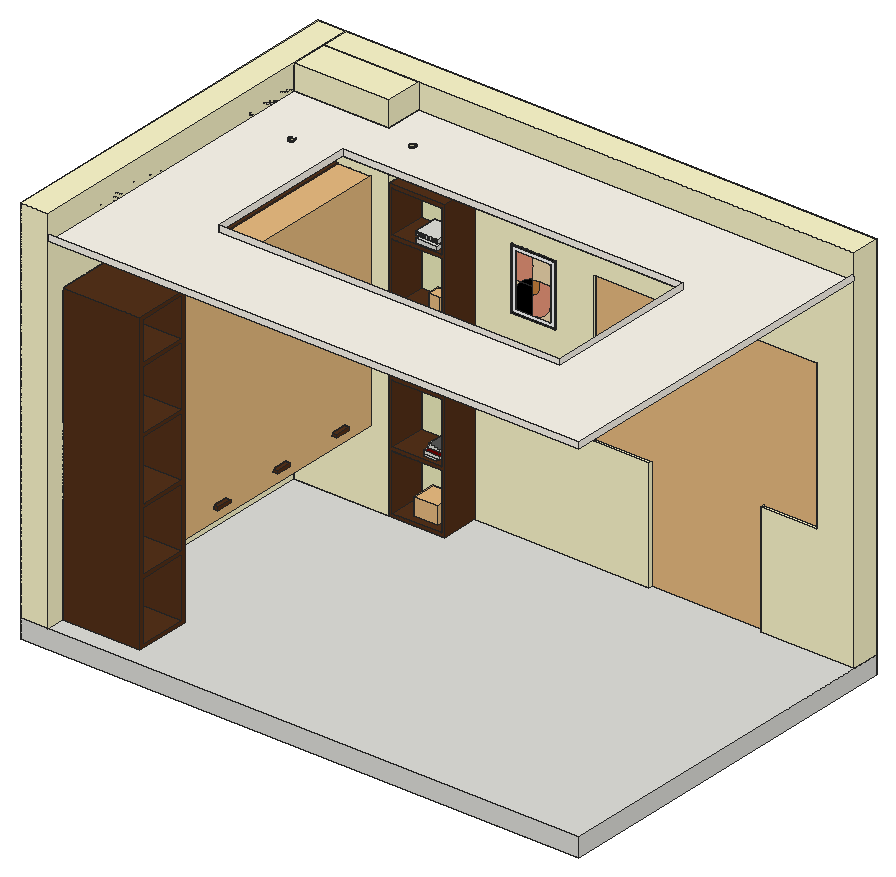
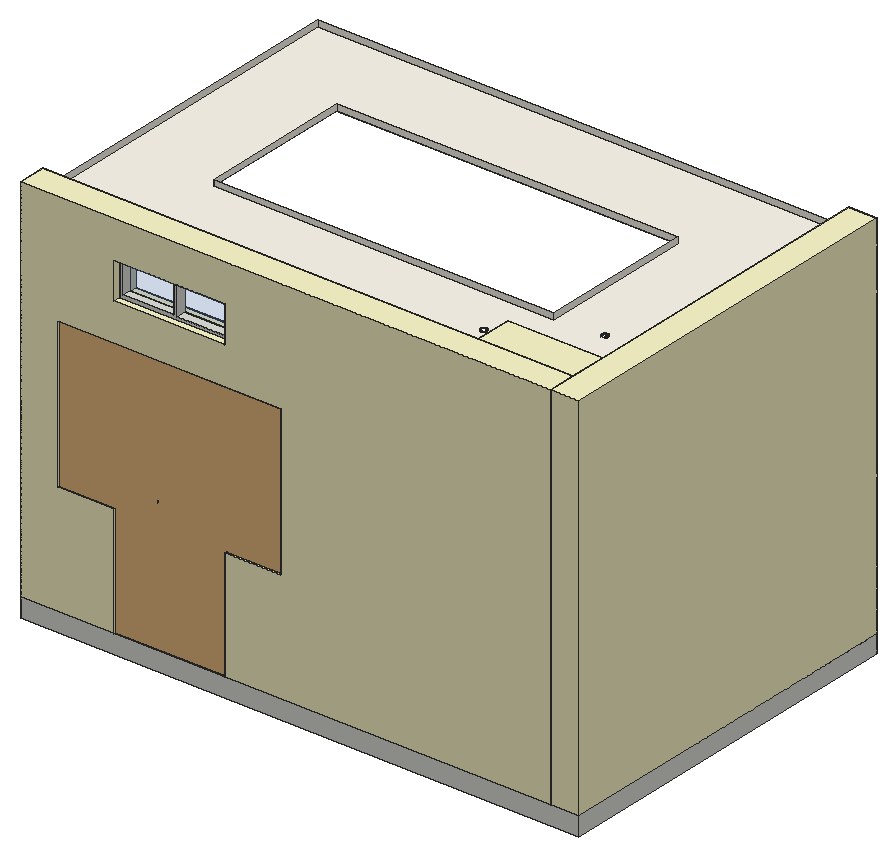
# SketchUp Ruby script. Lengths in inches.
U = 1.inch
M = Sketchup.active_model
def pt(a) = Geom::Point3d.new(a.map { |v| v * U })
def face(e, loops, mat)
  f = e.add_face(loops[0].map { |a| pt(a) })
  loops[1..].each { |l| e.add_face(l.map { |a| pt(a) }).erase! }
  f.material = f.back_material = mat if mat
  f
end
# faces: each face lists its corners as indices into pts; further lists are holes
def faces(e, pts, list, mat = nil) = list.each { |f| face(e, (f[0].is_a?(Array) ? f : [f]).map { |l| l.map { |i| pts[i] } }, mat) }
# xy, xz, yz: faces in a plane at the given z, y or x. An outline is a flat list of corners, or four numbers for a rectangle; further outlines are holes
def ring(l) = l.size == 4 ? [[l[0], l[1]], [l[2], l[1]], [l[2], l[3]], [l[0], l[3]]] : l.each_slice(2).to_a
def flat(e, list, mat, &to3) = list.each { |f| face(e, (f[0].is_a?(Array) ? f : [f]).map { |l| ring(l).map { |u, v| to3.(u, v) } }, mat) }
def xy(e, z, list, mat = nil) = flat(e, list, mat) { |x, y| [x, y, z] }
def xz(e, y, list, mat = nil) = flat(e, list, mat) { |x, z| [x, y, z] }
def yz(e, x, list, mat = nil) = flat(e, list, mat) { |y, z| [x, y, z] }
def lines(e, pts, list) = list.each { |a, b| e.add_line(pt(pts[a]), pt(pts[b])) }
# prism: a flat outline (further loops are holes) pulled along v
def prism(e, loops, v, mat = nil)
  f = face(e, loops, mat); d = Geom::Vector3d.new(v.map { |x| x * U })
  f.pushpull(f.normal.samedirection?(d) ? d.length : -d.length)
end
def box(e, o, s, mat = nil) = prism(e, [[o, [o[0] + s[0], o[1], o[2]], [o[0] + s[0], o[1] + s[1], o[2]], [o[0], o[1] + s[1], o[2]]]], [0, 0, s[2]], mat)
def at(x, y, z, deg = 0) = Geom::Transformation.translation(pt([x, y, z])) * Geom::Transformation.rotation(ORIGIN, Z_AXIS, deg.degrees)
def axes(o, x, y, z) = Geom::Transformation.new([*x, 0, *y, 0, *z, 0, *pt(o).to_a, 1])
def part(name) = M.definitions.add(name)
# library, detail: a bought-in or finely detailed component or shape, given as its bounding box
def library(name, o, s) = part(name).tap { |d| box(d.entities, o, s) }
def detail(e, o, s) = box(e.add_group.entities, o, s)
def put(e, d, t, mat = nil) = e.add_instance(d, t).tap { |i| i.material = mat if mat }
def group(e, t, mat = nil) = e.add_group.tap { |g| g.transformation = t; g.material = mat if mat }.entities
root = M.entities
M.materials.add("[0014_DarkSalmon]").color = [233, 150, 122]
M.materials.add("[0034_Wheat]").color = [245, 222, 179]
M.materials.add("[0040_Peru]").color = [205, 133, 63]
M.materials.add("[0050_LemonChiffon]").color = [255, 250, 205]
M.materials.add("[0052_FloralWhite]").color = [255, 250, 240]
M.materials.add("[0137_Black]").color = [0, 0, 0]
M.materials.add("[Color A08]").color = [102, 0, 0]
M.materials.add("[Color D02]").color = [214, 192, 128]
M.materials.add("[Color D07]").color = [153, 114, 0]
M.materials.add("[Color E01]").color = [242, 242, 193]
M.materials.add("[Color E01]1").color = [255, 255, 204]
M.materials.add("[Color L16]").color = [102, 0, 51]
M.materials.add("[Color M00]").color = [255, 255, 255]
M.materials.add("[Color M06]").color = [86, 86, 86]
M.materials.add("[Color M07]").color = [58, 58, 58]
M.materials.add("[Color M09]").color = [0, 0, 0]
M.materials.add("[Metal Aluminum Anodized]").color = [202, 209, 219]
M.materials.add("[Translucent Glass Blue]").color = [107, 160, 255]
M.materials["[Translucent Glass Blue]"].alpha = 0.26
M.materials.add("[Translucent Glass Gray]").color = [128, 128, 128]
M.materials["[Translucent Glass Gray]"].alpha = 0.5
M.materials.add("[Wood Veneer 01]").color = [112, 65, 34]
M.materials.add("[Wood Veneer 01]1").color = [84, 49, 25]
c1 = library("Group\#12",[0,0,0],[72,7.3,84])
c2 = library("Group\#45",[0,0,0],[7.625,7.62,5.4375])
c3 = library("Group\#23",[2,0,0],[22.8,75,72])
c4 = part("Group\#31")
box(c4.entities,[0,0,0],[1.5,4.9375,1])
c5 = part("Group\#28")
box(c5.entities,[0,0,0],[1,1.53,44.5])
c6 = library("Group\#50",[0,0,0],[5.875,5.87,4.8125])
c7 = library("Group\#49",[0,0,0],[3.75,3.75,5.1875])
c8 = part("Group\#30")
box(c8.entities,[0,0,0],[1,0.5625,2.125])
box(root,[40.6,110.9,7],[16,0.1,94],"[Color E01]")
xy(root,118,[[[9,0,180,111],[39.6,30.6,149.4,80.4],[24.3,77.95,24.37,77.96,24.4375,77.96,24.51,77.98,24.58,77.99,24.64,78.01,24.71,78.04,24.77,78.07,24.83,78.11,24.89,78.14,24.94,78.1875,24.99,78.23,25.04,78.28,25.09,78.34,25.13,78.39,25.17,78.45,25.2,78.52,25.23,78.58,25.25,78.64,25.27,78.71,25.3,78.92,25.3,78.99,25.27,79.2,25.25,79.26,25.23,79.33,25.17,79.45,25.09,79.57,24.94,79.72,24.89,79.76,24.77,79.84,24.71,79.87,24.64,79.89,24.58,79.92,24.51,79.93,24.4375,79.94,24.37,79.95,24.23,79.95,24.02,79.92,23.96,79.89,23.89,79.87,23.83,79.84,23.71,79.76,23.66,79.72,23.51,79.57,23.43,79.45,23.37,79.33,23.35,79.26,23.33,79.2,23.3,78.99,23.3,78.92,23.33,78.71,23.35,78.64,23.37,78.58,23.4,78.52,23.43,78.45,23.47,78.39,23.51,78.34,23.56,78.28,23.61,78.23,23.66,78.1875,23.71,78.14,23.77,78.11,23.83,78.07,23.89,78.04,23.96,78.01,24.02,77.99,24.09,77.98,24.16,77.96,24.23,77.96],[49.94,94.53,50.15,94.53,50.29,94.55,50.36,94.5625,50.42,94.59,50.49,94.61,50.55,94.64,50.67,94.72,50.72,94.76,50.78,94.81,50.82,94.86,50.87,94.91,50.95,95.03,51.01,95.15,51.05,95.29,51.0625,95.35,51.07,95.42,51.08,95.49,51.08,95.5625,51.07,95.63,51.0625,95.7,51.05,95.77,51.03,95.84,51.01,95.9,50.98,95.97,50.94,96.03,50.91,96.09,50.87,96.14,50.82,96.2,50.77,96.25,50.72,96.29,50.66,96.34,50.61,96.375,50.55,96.41,50.48,96.44,50.42,96.47,50.35,96.49,50.28,96.5,50.22,96.52,50.01,96.52,49.9375,96.51,49.87,96.5,49.8,96.49,49.73,96.46,49.67,96.4375,49.61,96.41,49.43,96.29,49.33,96.19,49.29,96.14,49.21,96.02,49.15,95.9,49.11,95.76,49.09,95.7,49.08,95.63,49.08,95.42,49.09,95.35,49.13,95.21,49.15,95.15,49.18,95.08,49.21,95.02,49.25,94.96,49.29,94.91,49.34,94.85,49.39,94.8,49.4375,94.76,49.49,94.71,49.55,94.68,49.61,94.64,49.67,94.61,49.74,94.58,49.81,94.5625,49.875,94.55]]],"[0052_FloralWhite]")
xz(root,0,[[9,118,180,120]],"[0052_FloralWhite]")
xz(root,30.6,[[39.6,118,149.4,120]],"[0052_FloralWhite]")
xz(root,77.96,[[24.16,118,24.23,118.3],[24.37,118,24.4375,118.3]],"[Metal Aluminum Anodized]")
xz(root,80.4,[[39.6,118,149.4,120]],"[0052_FloralWhite]")
xz(root,94.53,[[49.94,118,50.01,118.125],[50.01,118,50.08,118.125],[50.08,118,50.15,118.125]],"[Metal Aluminum Anodized]")
xz(root,96.52,[[50.01,118,50.08,118.125],[50.08,118,50.15,118.125],[50.15,118,50.22,118.125]],"[Metal Aluminum Anodized]")
xz(root,114.5,[[115,103,131.5,113],[132.5,103,149,113]],"[Translucent Glass Blue]")
yz(root,9,[[0,118,111,120]],"[0052_FloralWhite]")
yz(root,23,[[82,40,98,101],[24.5,84.5,33.8125,101.5]],"[Translucent Glass Gray]")
yz(root,23.3,[[78.92,118,78.99,118.3]],"[Metal Aluminum Anodized]")
yz(root,25.3,[[78.92,118,78.99,118.3]],"[Metal Aluminum Anodized]")
yz(root,39.6,[[30.6,118,80.4,120]],"[0052_FloralWhite]")
yz(root,49.08,[[95.42,118,95.49,118.125],[95.49,118,95.56,118.125],[95.56,118,95.63,118.125]],"[Metal Aluminum Anodized]")
yz(root,51.08,[[95.49,118,95.5625,118.125]],"[Metal Aluminum Anodized]")
yz(root,149.4,[[30.6,118,80.4,120]],"[0052_FloralWhite]")
yz(root,180,[[0,118,111,120]],"[0052_FloralWhite]")
p = [[23.89,78.04,118],[23.83,78.07,118],[23.83,78.07,118.3],[23.89,78.04,118.3],[23.96,78.01,118],[23.96,78.01,118.3],
  [24.09,77.98,118],[24.02,77.99,118],[24.02,77.99,118.3],[24.09,77.98,118.3],[24.16,77.96,118],[24.16,77.96,118.3],
  [24.3,77.95,118],[24.23,77.96,118],[24.23,77.96,118.3],[24.3,77.95,118.3],[24.37,77.96,118],[24.37,77.96,118.3],
  [24.51,77.98,118],[24.4375,77.96,118],[24.4375,77.96,118.3],[24.51,77.98,118.3],[24.58,77.99,118],[24.58,77.99,118.3],
  [24.71,78.04,118],[24.64,78.01,118],[24.64,78.01,118.3],[24.71,78.04,118.3],[24.77,78.07,118],[24.77,78.07,118.3],
  [23.77,78.11,118],[23.71,78.14,118],[23.71,78.14,118.3],[23.77,78.11,118.3],[23.66,78.1875,118],[23.66,78.1875,118.3],
  [24.89,78.14,118],[24.83,78.11,118],[24.83,78.11,118.3],[24.89,78.14,118.3],[24.94,78.1875,118],[24.94,78.1875,118.3],
  [23.61,78.23,118],[23.61,78.23,118.3],[23.56,78.28,118],[23.56,78.28,118.3],[24.99,78.23,118],[24.99,78.23,118.3],
  [25.04,78.28,118],[25.04,78.28,118.3],[23.51,78.34,118],[23.51,78.34,118.3],[23.47,78.39,118],[23.47,78.39,118.3],
  [25.09,78.34,118],[25.09,78.34,118.3],[25.13,78.39,118],[25.13,78.39,118.3],[23.43,78.45,118],[23.43,78.45,118.3],
  [25.17,78.45,118],[25.17,78.45,118.3],[23.4,78.52,118],[23.4,78.52,118.3],[23.37,78.58,118],[23.37,78.58,118.3],
  [25.23,78.58,118],[25.2,78.52,118],[25.2,78.52,118.3],[25.23,78.58,118.3],[23.35,78.64,118],[23.35,78.64,118.3],
  [23.33,78.71,118],[23.33,78.71,118.3],[25.25,78.64,118],[25.25,78.64,118.3],[25.27,78.71,118],[25.27,78.71,118.3],
  [23.32,78.78,118],[23.32,78.78,118.3],[25.28,78.78,118],[25.28,78.78,118.3],[23.31,78.85,118],[23.31,78.85,118.3],
  [23.3,78.92,118],[23.3,78.92,118.3],[25.3,78.92,118],[25.29,78.85,118],[25.29,78.85,118.3],[25.3,78.92,118.3],
  [23.3,78.99,118],[23.31,79.06,118],[23.31,79.06,118.3],[23.3,78.99,118.3],[25.29,79.06,118],[25.3,78.99,118],
  [25.3,78.99,118.3],[25.29,79.06,118.3],[23.32,79.13,118],[23.32,79.13,118.3],[23.33,79.2,118],[23.33,79.2,118.3],
  [25.27,79.2,118],[25.28,79.13,118],[25.28,79.13,118.3],[25.27,79.2,118.3],[23.35,79.26,118],[23.35,79.26,118.3],
  [25.25,79.26,118],[25.25,79.26,118.3],[23.37,79.33,118],[23.37,79.33,118.3],[23.4,79.39,118],[23.4,79.39,118.3],
  [25.2,79.39,118],[25.23,79.33,118],[25.23,79.33,118.3],[25.2,79.39,118.3],[23.43,79.45,118],[23.43,79.45,118.3],
  [25.17,79.45,118],[25.17,79.45,118.3],[23.47,79.51,118],[23.47,79.51,118.3],[23.51,79.57,118],[23.51,79.57,118.3],
  [25.09,79.57,118],[25.13,79.51,118],[25.13,79.51,118.3],[25.09,79.57,118.3],[23.56,79.62,118],[23.56,79.62,118.3],
  [23.61,79.67,118],[23.61,79.67,118.3],[24.99,79.67,118],[25.04,79.62,118],[25.04,79.62,118.3],[24.99,79.67,118.3],
  [23.66,79.72,118],[23.66,79.72,118.3],[24.94,79.72,118],[24.94,79.72,118.3],[49.875,94.55,118],[49.81,94.5625,118],
  [49.81,94.5625,118.125],[49.875,94.55,118.125],[49.94,94.53,118],[49.94,94.53,118.125],[50.29,94.55,118],[50.22,94.54,118],
  [50.22,94.54,118.125],[50.29,94.55,118.125],[50.15,94.53,118],[50.15,94.53,118.125],[50.36,94.5625,118],[50.36,94.5625,118.125],
  [49.67,94.61,118],[49.61,94.64,118],[49.61,94.64,118.125],[49.67,94.61,118.125],[49.55,94.68,118],[49.55,94.68,118.125],
  [49.74,94.58,118],[49.74,94.58,118.125],[50.49,94.61,118],[50.42,94.59,118],[50.42,94.59,118.125],[50.49,94.61,118.125],
  [50.55,94.64,118],[50.55,94.64,118.125],[50.61,94.68,118],[50.61,94.68,118.125],[49.49,94.71,118],[49.4375,94.76,118],
  [49.4375,94.76,118.125],[49.49,94.71,118.125],[50.67,94.72,118],[50.67,94.72,118.125],[50.72,94.76,118],[50.72,94.76,118.125],
  [49.39,94.8,118],[49.34,94.85,118],[49.34,94.85,118.125],[49.39,94.8,118.125],[50.78,94.81,118],[50.78,94.81,118.125],
  [50.82,94.86,118],[50.82,94.86,118.125],[49.29,94.91,118],[49.29,94.91,118.125],[49.25,94.96,118],[49.25,94.96,118.125],
  [50.87,94.91,118],[50.87,94.91,118.125],[50.91,94.97,118],[50.91,94.97,118.125],[49.21,95.02,118],[49.21,95.02,118.125],
  [49.18,95.08,118],[49.18,95.08,118.125],[50.98,95.09,118],[50.95,95.03,118],[50.95,95.03,118.125],[50.98,95.09,118.125],
  [49.15,95.15,118],[49.13,95.21,118],[49.13,95.21,118.125],[49.15,95.15,118.125],[51.01,95.15,118],[51.01,95.15,118.125],
  [49.11,95.28,118],[49.11,95.28,118.125],[51.05,95.29,118],[51.03,95.22,118],[51.03,95.22,118.125],[51.05,95.29,118.125],
  [49.09,95.35,118],[49.09,95.35,118.125],[49.08,95.42,118],[49.08,95.42,118.125],[51.0625,95.35,118],[51.0625,95.35,118.125],
  [51.08,95.49,118],[51.07,95.42,118],[51.07,95.42,118.125],[51.08,95.49,118.125],[49.08,95.63,118],[49.09,95.7,118],
  [49.09,95.7,118.125],[49.08,95.63,118.125],[51.0625,95.7,118],[51.07,95.63,118],[51.07,95.63,118.125],[51.0625,95.7,118.125],
  [51.08,95.5625,118],[51.08,95.5625,118.125],[49.11,95.76,118],[49.11,95.76,118.125],[51.05,95.77,118],[51.05,95.77,118.125],
  [49.13,95.83,118],[49.13,95.83,118.125],[49.15,95.9,118],[49.15,95.9,118.125],[51.01,95.9,118],[51.03,95.84,118],
  [51.03,95.84,118.125],[51.01,95.9,118.125],[49.18,95.96,118],[49.18,95.96,118.125],[50.98,95.97,118],[50.98,95.97,118.125],
  [49.21,96.02,118],[49.21,96.02,118.125],[49.25,96.08,118],[49.25,96.08,118.125],[50.91,96.09,118],[50.94,96.03,118],
  [50.94,96.03,118.125],[50.91,96.09,118.125],[49.29,96.14,118],[49.29,96.14,118.125],[49.33,96.19,118],[49.33,96.19,118.125],
  [50.82,96.2,118],[50.87,96.14,118],[50.87,96.14,118.125],[50.82,96.2,118.125],[49.38,96.24,118],[49.38,96.24,118.125],
  [49.43,96.29,118],[49.43,96.29,118.125],[50.72,96.29,118],[50.77,96.25,118],[50.77,96.25,118.125],[50.72,96.29,118.125],
  [49.49,96.33,118],[49.49,96.33,118.125],[49.55,96.37,118],[49.55,96.37,118.125],[50.61,96.375,118],[50.66,96.34,118],
  [50.66,96.34,118.125],[50.61,96.375,118.125],[49.61,96.41,118],[49.61,96.41,118.125],[49.67,96.4375,118],[49.67,96.4375,118.125],
  [49.73,96.46,118],[49.73,96.46,118.125],[50.42,96.47,118],[50.48,96.44,118],[50.48,96.44,118.125],[50.42,96.47,118.125],
  [50.55,96.41,118],[50.55,96.41,118.125],[49.8,96.49,118],[49.8,96.49,118.125],[49.87,96.5,118],[49.87,96.5,118.125],
  [49.9375,96.51,118],[49.9375,96.51,118.125],[50.01,96.52,118],[50.01,96.52,118.125],[50.22,96.52,118],[50.28,96.5,118],
  [50.28,96.5,118.125],[50.22,96.52,118.125],[50.35,96.49,118],[50.35,96.49,118.125],[27.57,69.71,39],[27.57,65.4,39],
  [31.38,65.4,39],[31.38,69.71,39],[49.62,102.35,27.76],[53.375,102.35,27.76]]
faces(root,p,[[0,1,2,3],[4,0,3,5],[6,7,8,9],[7,4,5,8],[10,6,9,11],[12,13,14,15],[16,12,15,17],[18,19,20,21],
  [22,18,21,23],[24,25,26,27],[25,22,23,26],[28,24,27,29],[30,31,32,33],[31,34,35,32],[1,30,33,2],[36,37,38,39],
  [37,28,29,38],[40,36,39,41],[34,42,43,35],[42,44,45,43],[46,40,41,47],[48,46,47,49],[44,50,51,45],[50,52,53,51],
  [54,48,49,55],[56,54,55,57],[52,58,59,53],[60,56,57,61],[58,62,63,59],[62,64,65,63],[66,67,68,69],[67,60,61,68],
  [64,70,71,65],[70,72,73,71],[74,66,69,75],[76,74,75,77],[72,78,79,73],[80,76,77,81],[78,82,83,79],[82,84,85,83],
  [86,87,88,89],[87,80,81,88],[90,91,92,93],[94,95,96,97],[91,98,99,92],[98,100,101,99],[102,103,104,105],[103,94,97,104],
  [100,106,107,101],[108,102,105,109],[106,110,111,107],[110,112,113,111],[114,115,116,117],[115,108,109,116],[112,118,119,113],[120,114,117,121],
  [118,122,123,119],[122,124,125,123],[126,127,128,129],[127,120,121,128],[124,130,131,125],[130,132,133,131],[134,135,136,137],[135,126,129,136],
  [132,138,139,133],[140,134,137,141],[142,143,144,145],[146,142,145,147],[148,149,150,151],[149,152,153,150],[154,148,151,155],[156,157,158,159],
  [157,160,161,158],[143,162,163,144],[162,156,159,163],[164,165,166,167],[165,154,155,166],[168,164,167,169],[170,168,169,171],[172,173,174,175],
  [160,172,175,161],[176,170,171,177],[178,176,177,179],[180,181,182,183],[173,180,183,174],[184,178,179,185],[186,184,185,187],[181,188,189,182],
  [188,190,191,189],[192,186,187,193],[194,192,193,195],[190,196,197,191],[196,198,199,197],[200,201,202,203],[201,194,195,202],[204,205,206,207],
  [198,204,207,199],[208,200,203,209],[205,210,211,206],[212,213,214,215],[213,208,209,214],[210,216,217,211],[216,218,219,217],[220,212,215,221],
  [222,223,224,225],[223,220,221,224],[226,227,228,229],[230,231,232,233],[231,234,235,232],[227,236,237,228],[238,230,233,239],[236,240,241,237],
  [240,242,243,241],[244,245,246,247],[245,238,239,246],[242,248,249,243],[250,244,247,251],[248,252,253,249],[252,254,255,253],[256,257,258,259],
  [257,250,251,258],[254,260,261,255],[260,262,263,261],[264,265,266,267],[265,256,259,266],[262,268,269,263],[268,270,271,269],[272,273,274,275],
  [273,264,267,274],[270,276,277,271],[276,278,279,277],[280,281,282,283],[281,272,275,282],[278,284,285,279],[284,286,287,285],[286,288,289,287],
  [290,291,292,293],[291,294,295,292],[294,280,283,295],[288,296,297,289],[296,298,299,297],[298,300,301,299],[300,302,303,301],[304,305,306,307],
  [305,308,309,306],[308,290,293,309]],"[Metal Aluminum Anodized]")
lines(root,p,[[310,311],[311,312],[312,313],[313,310],[314,315]])
g1 = group(root,at(0,0,0))
box(g1,[0,0,0],[180,120,6])
g2 = group(root,at(9,6,6),"[Wood Veneer 01]1")
xy(g2,0,[[0,0,24.8,18]])
xy(g2,1,[[0,1,24.8,17]])
xy(g2,20.2,[[0,1,24.8,17]])
xy(g2,21.2,[[0,1,24.8,17]])
xy(g2,40.6,[[0,1,24.8,17]])
xy(g2,41.6,[[0,1,24.8,17]])
xy(g2,61,[[0,1,24.8,17]])
xy(g2,62,[[0,1,24.8,17]])
xy(g2,78,[[2,18,14,27.8125]])
xy(g2,78.1,[[2,18,14,18,14,18.5],[2,18,14,18.5,14,27.8125,2,27.8125]],"[Wood Veneer 01]1")
xy(g2,81.4,[[0,1,24.8,17]])
xy(g2,82.4,[[0,1,24.8,17]])
xy(g2,95,[[0,1,24.8,17]])
xy(g2,96,[[0,0,24.8,18]])
xz(g2,0,[[0,0,24.8,96]])
xz(g2,1,[[0,1,24.8,20.2],[0,21.2,24.8,40.6],[0,41.6,24.8,61],[0,62,24.8,81.4],[0,82.4,24.8,95]])
xz(g2,17,[[0,1,24.8,20.2],[0,21.2,24.8,40.6],[0,41.6,24.8,61],[0,62,24.8,81.4],[0,82.4,24.8,95]])
xz(g2,18,[[0,0,0,96,24.8,96,24.8,78.1,2,78.1,2,78,24.8,78,24.8,0],[2,78,14,78.1],[14,78,24.8,78.1]])
xz(g2,27.8125,[[2,78,14,78.1]])
yz(g2,0,[[[0,0,18,96],[1,62,17,81.4],[1,41.6,17,61],[1,21.2,17,40.6],[1,1,17,20.2],[1,82.4,17,95]]])
yz(g2,2,[[18,78,27.8125,78.1]])
yz(g2,14,[[18,78,27.8125,78.1]])
yz(g2,24.8,[[[0,0,18,96],[1,62,17,81.4],[1,41.6,17,61],[1,21.2,17,40.6],[1,1,17,20.2],[1,82.4,17,95]]])
p = [[14,18.5,78.1],[14,18.5,95.5],[2,18,95.5],[2,18,78.1],[14,27.8125,78.1],[14,27.8125,95.5]]
faces(g2,p,[[0,1,2,3]],"[Wood Veneer 01]1")
lines(g2,p,[[4,5],[5,1]])
g3 = group(root,at(9,111,6),"[0050_LemonChiffon]")
prism(g3,[[[105,9,0],[0,9,0],[0,9,120],[171,9,120],[171,9,0],[141,9,0],[141,9,36],[159,9,36],[159,9,84],[141,9,84],[105,9,84],[87,9,84],[87,9,36],[105,9,36]],[[105,9,108],[105,9,96],[141,9,96],[141,9,108]]],[0,-9,0])
put(root,c1,at(96,112.1,6),"[Wood Veneer 01]")
g4 = group(root,at(0,0,6),"[0050_LemonChiffon]")
box(g4,[0,0,0],[9,120,120])
g5 = group(root,at(9,99,6),"[0050_LemonChiffon]")
xy(g5,0,[[0,0,30.6,12]])
xy(g5,120,[[0,0,30.6,12]])
xz(g5,0,[[0,0,30.6,112],[0,112,30.6,120]])
xz(g5,12,[[0,0,30.6,120]])
yz(g5,0,[[0,0,12,120]])
yz(g5,30.6,[[0,0,12,112],[0,112,12,120]])
g6 = group(root,at(39.6,99,6),"[Wood Veneer 01]1")
prism(g6,[[[0,12,0],[0,12,96],[18,12,96],[18,12,0]],[[1,12,61],[17,12,61],[17,12,80.4],[1,12,80.4]],[[1,12,40.6],[17,12,40.6],[17,12,60],[1,12,60]],[[1,12,39.6],[1,12,20.2],[17,12,20.2],[17,12,39.6]],[[17,12,19.2],[1,12,19.2],[1,12,1],[17,12,1]],[[1,12,95],[1,12,81.4],[17,12,81.4],[17,12,95]]],[0,-12,0])
put(root,c2,at(45.72,101.62,7))
g7 = group(root,at(49.62,100.4375,26.2))
box(g7,[0,0,0],[4.375,9.5625,0.625])
g8 = group(root,at(49.62,100.4375,26.83))
xy(g8,0,[[0,0,5.19,7.98]])
xy(g8,0.9375,[[0,0,5.19,7.98]],"[Color A08]")
xz(g8,0,[[0,0,5.19,0.9375]])
xz(g8,7.98,[[0,0,5.19,0.9375]])
yz(g8,0,[[0,0,7.98,0.9375]])
yz(g8,5.19,[[0,0,7.98,0.9375]])
g9 = group(root,at(49.62,102.35,26.98))
xz(g9,0,[[3.58,0,3.89,1.4,0.31,2.19,0,0.79]])
xz(g9,6.74,[[3.58,0,0,0.79,0.31,2.19,3.89,1.4]])
p = [[0,6.74,0.79],[3.58,6.74,0],[3.58,0,0],[0,0,0.79],[3.89,6.74,1.4],[3.89,0,1.4],
  [0.31,0,2.19],[0.31,6.74,2.19]]
faces(g9,p,[[0,1,2,3],[2,1,4,5],[0,3,6,7]])
faces(g9,p,[[4,7,6,5]],"[Color M06]")
put(root,c3,at(9,24,30))
put(root,c4,at(33.8,35.63,33.77),"[Wood Veneer 01]1")
put(root,c4,at(33.8,59.7,33.77),"[Wood Veneer 01]1")
put(root,c4,at(33.8,83.45,33.77),"[Wood Veneer 01]1")
g10 = group(root,at(21,44.2,39))
box(g10,[4.625,0,0],[4.6875,15.58,0.91])
g11 = group(g10,at(0.17,0.22,1.97))
xy(g11,0,[[0,0,0.5,18.23]])
xy(g11,1.49,[[0,0,0.5,18.23]])
xy(g11,12.08,[[0,0,0.5,18.23]])
xz(g11,0,[[0,0,0.5,1.49],[0,1.49,0.5,12.08]])
xz(g11,18.23,[[0,0,0.5,1.49],[0,1.49,0.5,12.08]])
yz(g11,0,[[0,0,18.23,1.49],[0,1.49,18.23,12.08]])
yz(g11,0.5,[[0,0,18.23,1.49]])
yz(g11,0.5,[[0,1.49,18.23,12.08]],"[Color M09]")
g12 = group(g10,at(0,6.74,0))
prism(g12,[[[0,0,0],[4.625,0,0],[4.625,0,0.29],[0.17,0,0.29],[0.17,0,2.78],[0,0,2.78]]],[0,2.65,0])
g13 = group(root,at(11,24,39),"[Color D02]")
put(g13,c5,at(0,4,0))
g14 = group(g13,at(0,0,0))
box(g14,[0,0.1875,0],[1,1.34,44.5])
put(g13,c5,at(0,2,0))
put(g13,c5,at(0,6,0))
put(g13,c5,at(0,56,0))
put(g13,c5,at(0,46,0))
put(g13,c5,at(0,44,0))
put(g13,c5,at(0,50,0))
put(g13,c5,at(0,54,0))
put(g13,c5,at(0,52,0))
put(g13,c5,at(0,48,0))
put(g13,c5,at(0,20,0))
put(g13,c5,at(0,34,0))
put(g13,c5,at(0,38,0))
put(g13,c5,at(0,40,0))
put(g13,c5,at(0,36,0))
put(g13,c5,at(0,18,0))
put(g13,c5,at(0,8,0))
put(g13,c5,at(0,14,0))
put(g13,c5,at(0,22,0))
put(g13,c5,at(0,26,0))
put(g13,c5,at(0,30,0))
put(g13,c5,at(0,12,0))
put(g13,c5,at(0,10,0))
put(g13,c5,at(0,24,0))
put(g13,c5,at(0,28,0))
put(g13,c5,at(0,16,0))
put(g13,c5,at(0,32,0))
put(g13,c5,at(0,42,0))
g15 = group(root,at(28.74,65.68,39))
xy(g15,0,[[0.92,0,0,1.08,1.36,2.94,2.28,1.87]])
p = [[0.07,1.17,0.19],[0,1.08,0],[0.92,0,0],[0.98,0.09,0.19],[2.28,1.87,0],[2.21,1.78,0.19],
  [2.12,1.65,0.36],[2.01,1.5,0.5],[1.88,1.32,0.6],[1.74,1.13,0.67],[1.6,0.93,0.6875],[1.45,0.73,0.67],
  [1.3125,0.54,0.6],[1.18,0.37,0.5],[1.07,0.21,0.36],[0.16,1.29,0.36],[0.27,1.44,0.5],[0.39,1.62,0.6],
  [0.53,1.8125,0.67],[0.68,2.01,0.6875],[0.82,2.21,0.67],[0.96,2.4,0.6],[1.09,2.58,0.5],[1.2,2.73,0.36],
  [1.29,2.85,0.19],[1.36,2.94,0]]
faces(g15,p,[[0,1,2,3],[3,2,4,5,6,7,8,9,10,11,12,13,14],[1,0,15,16,17,18,19,20,21,22,23,24,25],[25,24,5,4],[15,0,3,14],[24,23,6,5],[16,15,14,13],[23,22,7,6],
  [17,16,13,12],[22,21,8,7],[18,17,12,11],[21,20,9,8],[19,18,11,10],[20,19,10,9]])
put(root,c6,at(17.89,70.03,39.01))
g16 = group(root,at(136.25,116,41.09))
xy(g16,0,[[7.3,0,8.67,1]])
xy(g16,1.09,[[7.86,0,8.01,1]])
xy(g16,7.02,[[7.625,1,7.625,2.0625,0,2.0625,0,3.125,8.25,3.125,8.25,1]])
xy(g16,8.4,[[7.625,1,8.25,1,8.25,3.125,0,3.125,0,2.0625,7.625,2.0625]])
xy(g16,10.0625,[[7.3,0,8.67,1]])
xz(g16,0,[[[7.3,0,8.67,10.0625],[7.86,1.09,7.72,1.14,7.6,1.22,7.5,1.32,7.43,1.45,7.4,1.6,7.41,1.74,7.45,1.88,7.53,2.01,7.64,2.11,7.77,2.17,7.91,2.21,8.06,2.2,8.2,2.16,8.32,2.08,8.42,1.97,8.49,1.84,8.52,1.69,8.51,1.55,8.47,1.41,8.39,1.28,8.28,1.18,8.15,1.12,8.01,1.09]]])
xz(g16,1,[[[7.3,0,8.67,10.0625],[7.86,1.09,8.01,1.09,8.15,1.12,8.28,1.18,8.39,1.28,8.47,1.41,8.51,1.55,8.52,1.69,8.49,1.84,8.42,1.97,8.32,2.08,8.2,2.16,8.06,2.2,7.91,2.21,7.77,2.17,7.64,2.11,7.53,2.01,7.45,1.88,7.41,1.74,7.4,1.6,7.43,1.45,7.5,1.32,7.6,1.22,7.72,1.14],[7.625,7.02,8.25,8.4]]])
xz(g16,2.0625,[[0,7.02,7.625,8.4]])
xz(g16,3.125,[[0,7.02,8.25,8.4]])
yz(g16,0,[[2.0625,7.02,3.125,8.4]])
yz(g16,7.3,[[0,0,1,10.0625]])
yz(g16,7.625,[[1,7.02,2.0625,8.4]])
yz(g16,8.25,[[1,7.02,3.125,8.4]])
yz(g16,8.67,[[0,0,1,10.0625]])
p = [[7.72,1,1.14],[7.6,1,1.22],[7.6,0,1.22],[7.72,0,1.14],[7.86,1,1.09],[7.86,0,1.09],
  [8.15,1,1.12],[8.01,1,1.09],[8.01,0,1.09],[8.15,0,1.12],[8.28,1,1.18],[8.28,0,1.18],
  [7.5,1,1.32],[7.5,0,1.32],[8.39,1,1.28],[8.39,0,1.28],[7.43,1,1.45],[7.43,0,1.45],
  [8.47,1,1.41],[8.47,0,1.41],[8.51,1,1.55],[8.51,0,1.55],[7.4,1,1.6],[7.4,0,1.6],
  [8.52,1,1.69],[8.52,0,1.69],[7.41,1,1.74],[7.41,0,1.74],[7.45,1,1.88],[7.45,0,1.88],
  [8.49,1,1.84],[8.49,0,1.84],[8.42,1,1.97],[8.42,0,1.97],[7.53,1,2.01],[7.53,0,2.01],
  [7.64,1,2.11],[7.64,0,2.11],[8.32,1,2.08],[8.32,0,2.08],[7.77,1,2.17],[7.77,0,2.17],
  [8.2,1,2.16],[8.2,0,2.16],[7.91,1,2.21],[7.91,0,2.21],[8.06,1,2.2],[8.06,0,2.2]]
faces(g16,p,[[0,1,2,3],[4,0,3,5],[6,7,8,9],[10,6,9,11],[1,12,13,2],[14,10,11,15],[12,16,17,13],[18,14,15,19],
  [20,18,19,21],[16,22,23,17],[24,20,21,25],[22,26,27,23],[26,28,29,27],[30,24,25,31],[32,30,31,33],[28,34,35,29],
  [34,36,37,35],[38,32,33,39],[36,40,41,37],[42,38,39,43],[40,44,45,41],[44,46,47,45],[46,42,43,47]])
g17 = group(root,at(69.6,110.7,42),"[0034_Wheat]")
xy(g17,0,[[0,0,14.4,0.3]],"[Color E01]1")
xy(g17,0.3,[[0.3,0,14.1,0.1],[0.3,0.1,14.1,0.3]],"[Color E01]1")
xy(g17,1.6,[[1.6,0,12.8,0.1]],"[Color E01]1")
xy(g17,18.4,[[1.6,0,12.8,0.1]],"[Color E01]1")
xy(g17,19.7,[[0.3,0,14.1,0.1],[0.3,0.1,14.1,0.3]],"[Color E01]1")
xy(g17,20,[[0,0,14.4,0.3]],"[Color E01]1")
xz(g17,0,[[8.04,1.6,8.04,10,8.64,9.46,9.15,8.83,9.56,8.14,9.86,7.39,10.04,6.6,10.1,5.8,10.04,5,9.86,4.21,9.56,3.46,9.15,2.77,8.64,2.14],[1.6,10,8.04,18.4]],"[0034_Wheat]")
xz(g17,0,[[8.04,10,8.04,18.4,12.8,18.4,12.8,11.49,12.75,11.29,12.68,11.09,12.59,10.9,12.48,10.73,12.34,10.57,12.19,10.42,12.03,10.3,11.84,10.19,11.65,10.11,11.45,10.05,11.25,10.01,11.04,10]],"[0137_Black]")
xz(g17,0,[[1.6,1.6,8.04,10]],"[Color A08]")
xz(g17,0,[[8.04,1.6,8.64,2.14,9.15,2.77,9.56,3.46,9.86,4.21,10.04,5,10.1,5.8,10.04,6.6,9.86,7.39,9.56,8.14,9.15,8.83,8.64,9.46,8.04,10,11.04,10,11.25,10.01,11.45,10.05,11.65,10.11,11.84,10.19,12.03,10.3,12.19,10.42,12.34,10.57,12.48,10.73,12.59,10.9,12.68,11.09,12.75,11.29,12.8,11.49,12.8,1.6]],"[Color D07]")
xz(g17,0,[[[0,0,14.4,20],[0.3,0.3,14.1,19.7]]],"[Color M09]")
xz(g17,0.1,[[[0.3,0.3,14.1,19.7],[1.6,1.6,12.8,18.4]]],"[Color M00]")
xz(g17,0.3,[[[0,0,14.4,20],[0.3,0.3,14.1,19.7]]],"[Color E01]1")
yz(g17,0,[[0,0,0.3,20]],"[Color E01]1")
yz(g17,0.3,[[0,0.3,0.1,19.7],[0.1,0.3,0.3,19.7]],"[Color E01]1")
yz(g17,1.6,[[0,1.6,0.1,18.4]],"[Color E01]1")
yz(g17,12.8,[[0,1.6,0.1,18.4]],"[Color E01]1")
yz(g17,14.1,[[0,0.3,0.1,19.7],[0.1,0.3,0.3,19.7]],"[Color E01]1")
yz(g17,14.4,[[0,0,0.3,20]],"[Color E01]1")
g18 = group(root,at(40.6,102.03,46.6),"[Color M09]")
xy(g18,0,[[5.29,0,4.18,0.18,5.41,7.8,6.52,7.62],[4.18,0.18,2.5625,0.37,3.36,7.13,4.97,6.94],[0,0.37,2.5625,7.74]],"[Color M00]")
xy(g18,10.95,[[4.18,0.18,4.97,6.94,3.36,7.13,2.5625,0.37]],"[Color M00]")
xy(g18,11.9375,[[0,0.37,2.5625,7.74]],"[Color M00]")
xy(g18,12.39,[[5.29,0,6.52,7.62,5.41,7.8,4.18,0.18]],"[Color M00]")
xz(g18,0.37,[[[0,0,2.5625,11.9375],[0.69,1.07,2,11.07]]],"[Color M00]")
xz(g18,0.37,[[0.69,1.07,2,11.07]],"[Color M07]")
xz(g18,7.74,[[0,0,2.5625,11.9375]],"[Color M00]")
yz(g18,0,[[0.37,0,7.74,11.9375]],"[Color M00]")
yz(g18,2.5625,[[0.37,0,7.74,11.9375]],"[Color M00]")
p = [[4.18,0.18,10.95],[4.18,0.18,0],[5.29,0,0],[5.29,0,12.39],[4.18,0.18,12.39],[6.52,7.62,0],
  [6.52,7.62,12.39],[6.26,6.01,9.625],[6.26,6.01,2.125],[5.66,2.31,2.125],[5.66,2.31,9.625],[2.5625,0.37,10.95],
  [2.5625,0.37,0],[4.97,6.94,0],[4.97,6.94,10.95],[5.41,7.8,0],[5.41,7.8,12.39],[3.36,7.13,0],
  [3.36,7.13,10.95]]
faces(g18,p,[[0,1,2,3,4],[[2,5,6,3],[7,8,9,10]],[1,13,14,0],[15,1,0,4,16],[17,12,11,18],[17,18,14,13],[15,16,6,5]],"[Color M00]")
faces(g18,p,[[11,12,1,0]],"[Color M06]")
faces(g18,p,[[8,7,10,9]],"[Color L16]")
put(root,c7,at(49.48,102.62,67))
g19 = group(root,at(69.6,110.7,70))
xy(g19,0,[[0,0,14.4,0.3]])
xy(g19,0.3,[[0.3,0,14.1,0.1],[0.3,0.1,14.1,0.3]])
xy(g19,1.6,[[1.6,0,12.8,0.1]])
xy(g19,18.4,[[1.6,0,12.8,0.1]])
xy(g19,19.7,[[0.3,0,14.1,0.1],[0.3,0.1,14.1,0.3]])
xy(g19,20,[[0,0,14.4,0.3]])
xz(g19,0,[[7.2,1.6,7.2,7.94,7.48,7.93,7.75,7.97,8.02,8.04,8.27,8.15,8.51,8.3,8.72,8.48,8.9,8.69,9.05,8.93,9.16,9.18,9.23,9.45,9.27,9.72,9.26,10,9.26,12.06,12.8,12.06,12.8,5.93,12.71,5.48,12.44,4.72,12.06,4.01,11.5625,3.36,10.98,2.8,10.32,2.33,9.59,1.97,8.8125,1.72,8.02,1.6],[1.6,10,1.6,18.4,7.2,18.4,7.2,12.06,6.45,11.93,5.71,11.71,5.01,11.4,4.35,11.01,3.75,10.54,3.21,10]],"[0014_DarkSalmon]")
xz(g19,0,[[8.02,1.6,8.8125,1.72,9.59,1.97,10.32,2.33,10.98,2.8,11.5625,3.36,12.06,4.01,12.44,4.72,12.71,5.48,12.8,5.93,12.8,1.6],[1.6,5.8,1.6,10,3.21,10,3.2,10,2.73,9.4,2.33,8.74,2.01,8.05,1.79,7.32,1.65,6.5625],[7.2,12.06,12.8,18.4]],"[0034_Wheat]")
xz(g19,0,[[7.48,7.93,7.2,7.94,7.2,12.06,9.26,12.06,9.26,10,9.27,9.72,9.23,9.45,9.16,9.18,9.05,8.93,8.9,8.69,8.72,8.48,8.51,8.3,8.27,8.15,8.02,8.04,7.75,7.97]],"[0040_Peru]")
xz(g19,0,[[[0,0,14.4,20],[0.3,0.3,14.1,19.7]],[1.6,1.6,1.6,5.8,1.65,6.5625,1.79,7.32,2.01,8.05,2.33,8.74,2.73,9.4,3.2,10,7.2,10,7.2,1.6],[3.21,10,3.75,10.54,4.35,11.01,5.01,11.4,5.71,11.71,6.45,11.93,7.2,12.06,7.2,10]],"[Color M09]")
xz(g19,0.1,[[[0.3,0.3,14.1,19.7],[1.6,1.6,12.8,18.4]]],"[Color M00]")
xz(g19,0.3,[[[0,0,14.4,20],[0.3,0.3,14.1,19.7]]])
yz(g19,0,[[0,0,0.3,20]])
yz(g19,0.3,[[0,0.3,0.1,19.7],[0.1,0.3,0.3,19.7]])
yz(g19,1.6,[[0,1.6,0.1,18.4]])
yz(g19,12.8,[[0,1.6,0.1,18.4]])
yz(g19,14.1,[[0,0.3,0.1,19.7],[0.1,0.3,0.3,19.7]])
yz(g19,14.4,[[0,0,0.3,20]])
g20 = group(root,at(15.6,64.88,72))
detail(g20,[0,0,0],[5.375,5.375,2.8125])
g21 = group(root,at(11,24,83.5),"[Wood Veneer 01]1")
box(g21,[0,0,0],[12,57,0.5])
put(root,c8,at(23,69.49,86.1),"[Wood Veneer 01]1")
put(root,c8,at(23,67.49,86.1),"[Wood Veneer 01]1")
put(root,c8,at(23,44.86,86.1),"[Wood Veneer 01]1")
put(root,c8,at(23,42.74,86.1),"[Wood Veneer 01]1")
g22 = group(root,at(47.66,99.78,87.4))
box(g22,[0,0,0],[6.9375,9.75,1.1875])
g23 = group(root,at(47.66,101.36,88.59))
box(g23,[0,0,0],[6.9375,6.1,1])
g24 = group(root,at(47.66,99.8,89.59))
xy(g24,0,[[0,-0.125,7.25,7.67]])
xy(g24,0.08,[[0.2,-0.125,7.25,0.1]])
xy(g24,0.16,[[0.2,-0.125,7.25,0.1]])
xy(g24,0.23,[[0.2,-0.125,7.25,-0.1]])
xy(g24,0.31,[[0.2,-0.125,7.25,-0.1]])
xy(g24,0.38,[[0.2,-0.125,7.25,-0.1]])
xy(g24,0.46,[[0.2,-0.125,7.25,-0.1]])
xy(g24,0.53,[[0.2,-0.125,7.25,-0.1]])
xy(g24,0.61,[[0.2,-0.125,7.25,-0.1]])
xy(g24,0.68,[[0.2,-0.125,7.25,-0.1]])
xy(g24,0.76,[[0.2,-0.125,7.25,-0.1]])
xy(g24,0.83,[[0.2,-0.125,7.25,-0.1]])
xy(g24,0.91,[[0.2,-0.125,7.25,-0.1]])
xy(g24,0.98,[[0.2,-0.125,7.25,-0.1]])
xy(g24,1.06,[[0.2,-0.125,7.25,-0.1]])
xy(g24,1.13,[[0.2,-0.125,7.25,-0.1]])
xy(g24,1.21,[[0.2,-0.125,7.25,-0.1]])
xy(g24,1.25,[[0,-0.125,7.25,7.67]])
xz(g24,-0.125,[[0,0,7.25,0,7.25,0.08,0.2,0.08,0.2,0.16,7.25,0.16,7.25,0.23,0.2,0.23,0.2,0.31,7.25,0.31,7.25,0.38,0.2,0.38,0.2,0.46,7.25,0.46,7.25,0.53,0.2,0.53,0.2,0.61,7.25,0.61,7.25,0.68,0.2,0.68,0.2,0.76,7.25,0.76,7.25,0.83,0.2,0.83,0.2,0.91,7.25,0.91,7.25,0.98,0.2,0.98,0.2,1.06,7.25,1.06,7.25,1.13,0.2,1.13,0.2,1.21,7.25,1.21,7.25,1.25,0,1.25]])
xz(g24,-0.1,[[0.2,0.23,7.25,0.31],[0.2,0.38,7.25,0.46],[0.2,0.53,7.25,0.61],[0.2,0.68,7.25,0.76],[0.2,0.83,7.25,0.91],
  [0.2,0.98,7.25,1.06],[0.2,1.13,7.25,1.21]])
xz(g24,0.1,[[0.2,0.08,7.25,0.16]])
xz(g24,7.67,[[0,0,7.25,1.25]])
yz(g24,0,[[-0.125,0,7.67,1.25]])
yz(g24,0.2,[[-0.125,0.08,0.1,0.16],[-0.125,0.23,-0.1,0.31],[-0.125,0.38,-0.1,0.46],[-0.125,0.53,-0.1,0.61],[-0.125,0.68,-0.1,0.76],
  [-0.125,0.83,-0.1,0.91],[-0.125,0.98,-0.1,1.06],[-0.125,1.13,-0.1,1.21]])
yz(g24,7.25,[[-0.125,0,7.67,0,7.67,1.25,-0.125,1.25,-0.125,1.21,-0.1,1.21,-0.1,1.13,-0.125,1.13,-0.125,1.06,-0.1,1.06,-0.1,0.98,-0.125,0.98,-0.125,0.91,-0.1,0.91,-0.1,0.83,-0.125,0.83,-0.125,0.76,-0.1,0.76,-0.1,0.68,-0.125,0.68,-0.125,0.61,-0.1,0.61,-0.1,0.53,-0.125,0.53,-0.125,0.46,-0.1,0.46,-0.1,0.38,-0.125,0.38,-0.125,0.31,-0.1,0.31,-0.1,0.23,-0.125,0.23,-0.125,0.16,0.1,0.16,0.1,0.08,-0.125,0.08]])
g25 = group(root,at(114,115.5,102))
prism(g25,[[[0,-1,12],[0,-1,0],[36,-1,0],[36,-1,12]],[[17.5,-1,11],[17.5,-1,1],[1,-1,1],[1,-1,11]],[[18.5,-1,11],[35,-1,11],[35,-1,1],[18.5,-1,1]]],[0,3,0])
g26 = group(root,at(9,24,102),"[Wood Veneer 01]1")
box(g26,[0,0,0],[14.3,75,0.3])
